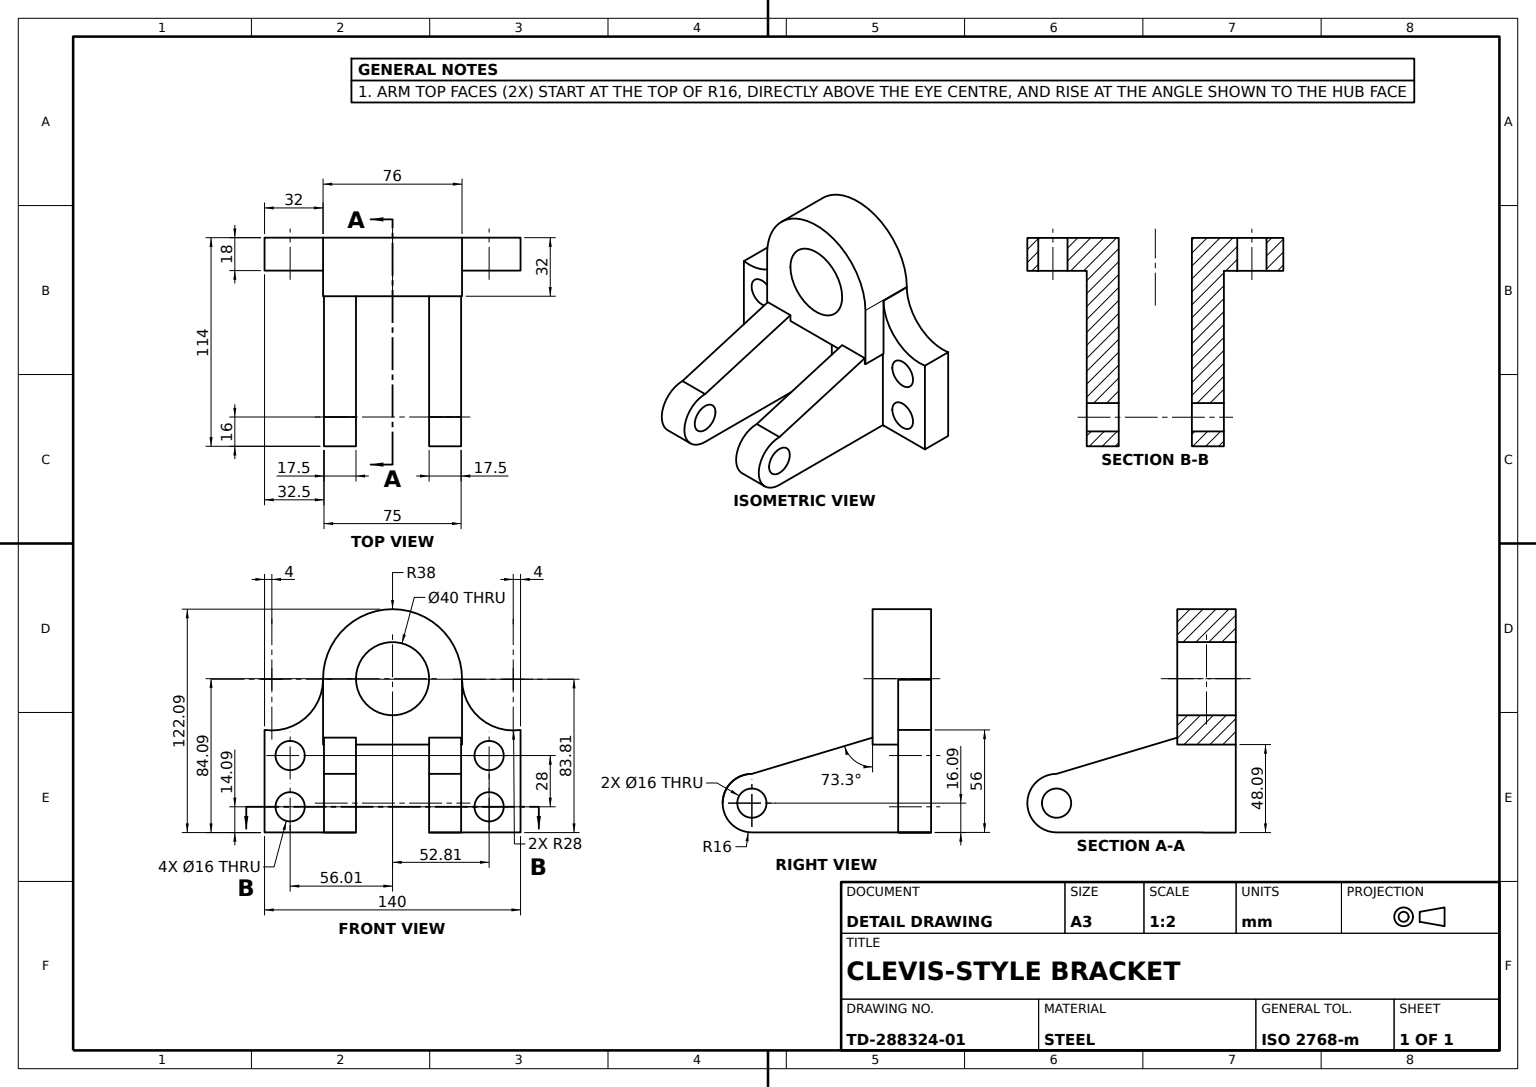
ISO-10303-21;
HEADER;
FILE_DESCRIPTION((''),'2;1');
FILE_NAME('','',(''),(''),'','','');
FILE_SCHEMA(('AUTOMOTIVE_DESIGN'));
ENDSEC;
DATA;
#1=APPLICATION_CONTEXT('');
#2=PRODUCT_CONTEXT('',#1,'mechanical');
#3=PRODUCT('','','',(#2));
#4=PRODUCT_DEFINITION_FORMATION('','',#3);
#5=PRODUCT_DEFINITION_CONTEXT('',#1,'design');
#6=PRODUCT_DEFINITION('','',#4,#5);
#7=PRODUCT_DEFINITION_SHAPE('','',#6);
#8=(LENGTH_UNIT()NAMED_UNIT(*)SI_UNIT(.MILLI.,.METRE.));
#9=(NAMED_UNIT(*)PLANE_ANGLE_UNIT()SI_UNIT($,.RADIAN.));
#10=(NAMED_UNIT(*)SI_UNIT($,.STERADIAN.)SOLID_ANGLE_UNIT());
#11=UNCERTAINTY_MEASURE_WITH_UNIT(LENGTH_MEASURE(1.E-05),#8,'distance_accuracy_value','');
#12=(GEOMETRIC_REPRESENTATION_CONTEXT(3)GLOBAL_UNCERTAINTY_ASSIGNED_CONTEXT((#11))GLOBAL_UNIT_ASSIGNED_CONTEXT((#8,#9,#10))REPRESENTATION_CONTEXT('',''));
#13=CARTESIAN_POINT('',(-48.006496,-34.,0.));
#14=VERTEX_POINT('',#13);
#15=CARTESIAN_POINT('',(-64.006496,-34.,0.));
#16=VERTEX_POINT('',#15);
#17=CARTESIAN_POINT('',(-56.006496,-34.,0.));
#18=DIRECTION('',(0.,0.,1.));
#19=DIRECTION('',(1.,0.,0.));
#20=AXIS2_PLACEMENT_3D('',#17,#18,#19);
#21=CIRCLE('',#20,8.);
#22=EDGE_CURVE('',#14,#16,#21,.T.);
#23=ORIENTED_EDGE('',*,*,#22,.F.);
#24=CARTESIAN_POINT('',(-48.006496,-34.,18.));
#25=VERTEX_POINT('',#24);
#26=VECTOR('',#18,1000.);
#27=LINE('',#13,#26);
#28=EDGE_CURVE('',#14,#25,#27,.T.);
#29=ORIENTED_EDGE('',*,*,#28,.T.);
#30=CARTESIAN_POINT('',(-64.006496,-34.,18.));
#31=VERTEX_POINT('',#30);
#32=CARTESIAN_POINT('',(-56.006496,-34.,18.));
#33=AXIS2_PLACEMENT_3D('',#32,#18,#19);
#34=CIRCLE('',#33,8.);
#35=EDGE_CURVE('',#25,#31,#34,.T.);
#36=ORIENTED_EDGE('',*,*,#35,.T.);
#37=LINE('',#15,#26);
#38=EDGE_CURVE('',#16,#31,#37,.T.);
#39=ORIENTED_EDGE('',*,*,#38,.F.);
#40=EDGE_LOOP('',(#23,#29,#36,#39));
#41=FACE_OUTER_BOUND('',#40,.T.);
#42=CYLINDRICAL_SURFACE('',#20,8.);
#43=ADVANCED_FACE('',(#41),#42,.F.);
#44=CARTESIAN_POINT('',(20.,-48.,98.));
#45=VERTEX_POINT('',#44);
#46=CARTESIAN_POINT('',(20.,-48.,18.));
#47=VERTEX_POINT('',#46);
#48=CARTESIAN_POINT('',(20.,-48.,114.));
#49=DIRECTION('',(0.,0.,-1.));
#50=VECTOR('',#49,1000.);
#51=LINE('',#48,#50);
#52=EDGE_CURVE('',#45,#47,#51,.T.);
#53=ORIENTED_EDGE('',*,*,#52,.T.);
#54=CARTESIAN_POINT('',(37.5,-48.,18.));
#55=VERTEX_POINT('',#54);
#56=DIRECTION('',(-1.,0.,0.));
#57=VECTOR('',#56,1000.);
#58=LINE('',#54,#57);
#59=EDGE_CURVE('',#55,#47,#58,.T.);
#60=ORIENTED_EDGE('',*,*,#59,.F.);
#61=CARTESIAN_POINT('',(37.5,-48.,98.));
#62=VERTEX_POINT('',#61);
#63=CARTESIAN_POINT('',(37.5,-48.,0.));
#64=LINE('',#63,#26);
#65=EDGE_CURVE('',#55,#62,#64,.T.);
#66=ORIENTED_EDGE('',*,*,#65,.T.);
#67=LINE('',#61,#57);
#68=EDGE_CURVE('',#62,#45,#67,.T.);
#69=ORIENTED_EDGE('',*,*,#68,.T.);
#70=EDGE_LOOP('',(#53,#60,#66,#69));
#71=FACE_OUTER_BOUND('',#70,.T.);
#72=DIRECTION('',(0.,-1.,0.));
#73=AXIS2_PLACEMENT_3D('',#63,#72,#49);
#74=PLANE('',#73);
#75=ADVANCED_FACE('',(#71),#74,.T.);
#76=CARTESIAN_POINT('',(-20.,-32.,90.));
#77=VERTEX_POINT('',#76);
#78=CARTESIAN_POINT('',(-20.,-32.,106.));
#79=VERTEX_POINT('',#78);
#80=CARTESIAN_POINT('',(-20.,-32.,98.));
#81=AXIS2_PLACEMENT_3D('',#80,#56,#72);
#82=CIRCLE('',#81,8.);
#83=EDGE_CURVE('',#77,#79,#82,.T.);
#84=ORIENTED_EDGE('',*,*,#83,.F.);
#85=CARTESIAN_POINT('',(-37.5,-32.,90.));
#86=VERTEX_POINT('',#85);
#87=CARTESIAN_POINT('',(70.,-32.,90.));
#88=LINE('',#87,#57);
#89=EDGE_CURVE('',#77,#86,#88,.T.);
#90=ORIENTED_EDGE('',*,*,#89,.T.);
#91=CARTESIAN_POINT('',(-37.5,-32.,106.));
#92=VERTEX_POINT('',#91);
#93=CARTESIAN_POINT('',(-37.5,-32.,98.));
#94=AXIS2_PLACEMENT_3D('',#93,#56,#18);
#95=CIRCLE('',#94,8.);
#96=EDGE_CURVE('',#86,#92,#95,.T.);
#97=ORIENTED_EDGE('',*,*,#96,.T.);
#98=CARTESIAN_POINT('',(70.,-32.,106.));
#99=LINE('',#98,#57);
#100=EDGE_CURVE('',#79,#92,#99,.T.);
#101=ORIENTED_EDGE('',*,*,#100,.F.);
#102=EDGE_LOOP('',(#84,#90,#97,#101));
#103=FACE_OUTER_BOUND('',#102,.T.);
#104=CARTESIAN_POINT('',(70.,-32.,98.));
#105=AXIS2_PLACEMENT_3D('',#104,#56,#18);
#106=CYLINDRICAL_SURFACE('',#105,8.);
#107=ADVANCED_FACE('',(#103),#106,.F.);
#108=CARTESIAN_POINT('',(37.5,-32.,90.));
#109=VERTEX_POINT('',#108);
#110=CARTESIAN_POINT('',(37.5,-32.,106.));
#111=VERTEX_POINT('',#110);
#112=CARTESIAN_POINT('',(37.5,-32.,98.));
#113=AXIS2_PLACEMENT_3D('',#112,#19,#49);
#114=CIRCLE('',#113,8.);
#115=EDGE_CURVE('',#109,#111,#114,.T.);
#116=ORIENTED_EDGE('',*,*,#115,.F.);
#117=EDGE_CURVE('',#111,#109,#114,.T.);
#118=ORIENTED_EDGE('',*,*,#117,.F.);
#119=EDGE_LOOP('',(#116,#118));
#120=FACE_BOUND('',#119,.T.);
#121=ORIENTED_EDGE('',*,*,#65,.F.);
#122=CARTESIAN_POINT('',(37.5,0.,18.));
#123=VERTEX_POINT('',#122);
#124=VECTOR('',#72,1000.);
#125=LINE('',#122,#124);
#126=EDGE_CURVE('',#123,#55,#125,.T.);
#127=ORIENTED_EDGE('',*,*,#126,.F.);
#128=CARTESIAN_POINT('',(37.5,0.,32.));
#129=VERTEX_POINT('',#128);
#130=LINE('',#128,#50);
#131=EDGE_CURVE('',#129,#123,#130,.T.);
#132=ORIENTED_EDGE('',*,*,#131,.F.);
#133=CARTESIAN_POINT('',(37.5,3.8,32.));
#134=VERTEX_POINT('',#133);
#135=CARTESIAN_POINT('',(37.5,36.,32.));
#136=DIRECTION('',(0.,1.,0.));
#137=VECTOR('',#136,1000.);
#138=LINE('',#135,#137);
#139=EDGE_CURVE('',#129,#134,#138,.T.);
#140=ORIENTED_EDGE('',*,*,#139,.T.);
#141=CARTESIAN_POINT('',(37.5,-16.,98.));
#142=VERTEX_POINT('',#141);
#143=CARTESIAN_POINT('',(37.5,12.293578,3.688073));
#144=DIRECTION('',(0.,0.287347886,-0.957826285));
#145=VECTOR('',#144,1000.);
#146=LINE('',#143,#145);
#147=EDGE_CURVE('',#142,#134,#146,.T.);
#148=ORIENTED_EDGE('',*,*,#147,.F.);
#149=CARTESIAN_POINT('',(37.5,-32.,114.));
#150=VERTEX_POINT('',#149);
#151=CIRCLE('',#113,16.);
#152=EDGE_CURVE('',#142,#150,#151,.T.);
#153=ORIENTED_EDGE('',*,*,#152,.T.);
#154=EDGE_CURVE('',#150,#62,#151,.T.);
#155=ORIENTED_EDGE('',*,*,#154,.T.);
#156=EDGE_LOOP('',(#121,#127,#132,#140,#148,#153,#155));
#157=FACE_OUTER_BOUND('',#156,.T.);
#158=CARTESIAN_POINT('',(37.5,0.,0.));
#159=AXIS2_PLACEMENT_3D('',#158,#19,#49);
#160=PLANE('',#159);
#161=ADVANCED_FACE('',(#120,#157),#160,.T.);
#162=CARTESIAN_POINT('',(-38.,-48.092936,18.));
#163=VERTEX_POINT('',#162);
#164=CARTESIAN_POINT('',(-38.,-48.092936,0.));
#165=VERTEX_POINT('',#164);
#166=LINE('',#162,#50);
#167=EDGE_CURVE('',#163,#165,#166,.T.);
#168=ORIENTED_EDGE('',*,*,#167,.F.);
#169=CARTESIAN_POINT('',(-38.,-48.,18.));
#170=VERTEX_POINT('',#169);
#171=CARTESIAN_POINT('',(-38.,0.,18.));
#172=LINE('',#171,#124);
#173=EDGE_CURVE('',#170,#163,#172,.T.);
#174=ORIENTED_EDGE('',*,*,#173,.F.);
#175=CARTESIAN_POINT('',(-38.,-48.,0.));
#176=VERTEX_POINT('',#175);
#177=LINE('',#169,#50);
#178=EDGE_CURVE('',#170,#176,#177,.T.);
#179=ORIENTED_EDGE('',*,*,#178,.T.);
#180=CARTESIAN_POINT('',(-38.,0.,0.));
#181=LINE('',#180,#124);
#182=EDGE_CURVE('',#176,#165,#181,.T.);
#183=ORIENTED_EDGE('',*,*,#182,.T.);
#184=EDGE_LOOP('',(#168,#174,#179,#183));
#185=FACE_OUTER_BOUND('',#184,.T.);
#186=AXIS2_PLACEMENT_3D('',#171,#19,#49);
#187=PLANE('',#186);
#188=ADVANCED_FACE('',(#185),#187,.F.);
#189=CARTESIAN_POINT('',(20.,-16.,98.));
#190=VERTEX_POINT('',#189);
#191=LINE('',#141,#57);
#192=EDGE_CURVE('',#142,#190,#191,.T.);
#193=ORIENTED_EDGE('',*,*,#192,.T.);
#194=CARTESIAN_POINT('',(20.,-32.,114.));
#195=VERTEX_POINT('',#194);
#196=CARTESIAN_POINT('',(20.,-32.,98.));
#197=AXIS2_PLACEMENT_3D('',#196,#19,#49);
#198=CIRCLE('',#197,16.);
#199=EDGE_CURVE('',#190,#195,#198,.T.);
#200=ORIENTED_EDGE('',*,*,#199,.T.);
#201=LINE('',#149,#57);
#202=EDGE_CURVE('',#150,#195,#201,.T.);
#203=ORIENTED_EDGE('',*,*,#202,.F.);
#204=ORIENTED_EDGE('',*,*,#152,.F.);
#205=EDGE_LOOP('',(#193,#200,#203,#204));
#206=FACE_OUTER_BOUND('',#205,.T.);
#207=AXIS2_PLACEMENT_3D('',#112,#56,#18);
#208=CYLINDRICAL_SURFACE('',#207,16.);
#209=ADVANCED_FACE('',(#206),#208,.T.);
#210=CARTESIAN_POINT('',(-20.,-48.,98.));
#211=VERTEX_POINT('',#210);
#212=CARTESIAN_POINT('',(-20.,-32.,114.));
#213=VERTEX_POINT('',#212);
#214=AXIS2_PLACEMENT_3D('',#80,#56,#18);
#215=CIRCLE('',#214,16.);
#216=EDGE_CURVE('',#211,#213,#215,.T.);
#217=ORIENTED_EDGE('',*,*,#216,.T.);
#218=CARTESIAN_POINT('',(-37.5,-32.,114.));
#219=VERTEX_POINT('',#218);
#220=EDGE_CURVE('',#213,#219,#201,.T.);
#221=ORIENTED_EDGE('',*,*,#220,.T.);
#222=CARTESIAN_POINT('',(-37.5,-48.,98.));
#223=VERTEX_POINT('',#222);
#224=AXIS2_PLACEMENT_3D('',#93,#19,#49);
#225=CIRCLE('',#224,16.);
#226=EDGE_CURVE('',#219,#223,#225,.T.);
#227=ORIENTED_EDGE('',*,*,#226,.T.);
#228=EDGE_CURVE('',#211,#223,#67,.T.);
#229=ORIENTED_EDGE('',*,*,#228,.F.);
#230=EDGE_LOOP('',(#217,#221,#227,#229));
#231=FACE_OUTER_BOUND('',#230,.T.);
#232=ADVANCED_FACE('',(#231),#208,.T.);
#233=CARTESIAN_POINT('',(70.,-48.,18.));
#234=VERTEX_POINT('',#233);
#235=CARTESIAN_POINT('',(70.,-48.,0.));
#236=VERTEX_POINT('',#235);
#237=LINE('',#233,#50);
#238=EDGE_CURVE('',#234,#236,#237,.T.);
#239=ORIENTED_EDGE('',*,*,#238,.F.);
#240=CARTESIAN_POINT('',(38.,-48.,18.));
#241=VERTEX_POINT('',#240);
#242=CARTESIAN_POINT('',(0.,-48.,18.));
#243=VECTOR('',#19,1000.);
#244=LINE('',#242,#243);
#245=EDGE_CURVE('',#241,#234,#244,.T.);
#246=ORIENTED_EDGE('',*,*,#245,.F.);
#247=CARTESIAN_POINT('',(38.,-48.,0.));
#248=VERTEX_POINT('',#247);
#249=LINE('',#240,#50);
#250=EDGE_CURVE('',#241,#248,#249,.T.);
#251=ORIENTED_EDGE('',*,*,#250,.T.);
#252=CARTESIAN_POINT('',(0.,-48.,0.));
#253=LINE('',#252,#243);
#254=EDGE_CURVE('',#248,#236,#253,.T.);
#255=ORIENTED_EDGE('',*,*,#254,.T.);
#256=EDGE_LOOP('',(#239,#246,#251,#255));
#257=FACE_OUTER_BOUND('',#256,.T.);
#258=AXIS2_PLACEMENT_3D('',#242,#136,#56);
#259=PLANE('',#258);
#260=ADVANCED_FACE('',(#257),#259,.F.);
#261=ORIENTED_EDGE('',*,*,#238,.T.);
#262=CARTESIAN_POINT('',(70.,8.,0.));
#263=VERTEX_POINT('',#262);
#264=CARTESIAN_POINT('',(70.,0.,0.));
#265=LINE('',#264,#137);
#266=EDGE_CURVE('',#236,#263,#265,.T.);
#267=ORIENTED_EDGE('',*,*,#266,.T.);
#268=CARTESIAN_POINT('',(70.,8.,18.));
#269=VERTEX_POINT('',#268);
#270=LINE('',#268,#50);
#271=EDGE_CURVE('',#269,#263,#270,.T.);
#272=ORIENTED_EDGE('',*,*,#271,.F.);
#273=CARTESIAN_POINT('',(70.,0.,18.));
#274=LINE('',#273,#137);
#275=EDGE_CURVE('',#234,#269,#274,.T.);
#276=ORIENTED_EDGE('',*,*,#275,.F.);
#277=EDGE_LOOP('',(#261,#267,#272,#276));
#278=FACE_OUTER_BOUND('',#277,.T.);
#279=AXIS2_PLACEMENT_3D('',#273,#56,#18);
#280=PLANE('',#279);
#281=ADVANCED_FACE('',(#278),#280,.F.);
#282=CARTESIAN_POINT('',(60.812643,-6.,18.));
#283=VERTEX_POINT('',#282);
#284=CARTESIAN_POINT('',(44.812643,-6.,18.));
#285=VERTEX_POINT('',#284);
#286=CARTESIAN_POINT('',(52.812643,-6.,18.));
#287=AXIS2_PLACEMENT_3D('',#286,#18,#19);
#288=CIRCLE('',#287,8.);
#289=EDGE_CURVE('',#283,#285,#288,.T.);
#290=ORIENTED_EDGE('',*,*,#289,.T.);
#291=CARTESIAN_POINT('',(44.812643,-6.,0.));
#292=VERTEX_POINT('',#291);
#293=LINE('',#291,#26);
#294=EDGE_CURVE('',#292,#285,#293,.T.);
#295=ORIENTED_EDGE('',*,*,#294,.F.);
#296=CARTESIAN_POINT('',(60.812643,-6.,0.));
#297=VERTEX_POINT('',#296);
#298=CARTESIAN_POINT('',(52.812643,-6.,0.));
#299=AXIS2_PLACEMENT_3D('',#298,#18,#19);
#300=CIRCLE('',#299,8.);
#301=EDGE_CURVE('',#297,#292,#300,.T.);
#302=ORIENTED_EDGE('',*,*,#301,.F.);
#303=LINE('',#296,#26);
#304=EDGE_CURVE('',#297,#283,#303,.T.);
#305=ORIENTED_EDGE('',*,*,#304,.T.);
#306=EDGE_LOOP('',(#290,#295,#302,#305));
#307=FACE_OUTER_BOUND('',#306,.T.);
#308=CYLINDRICAL_SURFACE('',#299,8.);
#309=ADVANCED_FACE('',(#307),#308,.F.);
#310=CARTESIAN_POINT('',(-37.5,-16.,98.));
#311=VERTEX_POINT('',#310);
#312=CARTESIAN_POINT('',(-37.5,3.8,32.));
#313=VERTEX_POINT('',#312);
#314=CARTESIAN_POINT('',(-37.5,12.293578,3.688073));
#315=LINE('',#314,#145);
#316=EDGE_CURVE('',#311,#313,#315,.T.);
#317=ORIENTED_EDGE('',*,*,#316,.F.);
#318=CARTESIAN_POINT('',(-20.,-16.,98.));
#319=VERTEX_POINT('',#318);
#320=EDGE_CURVE('',#319,#311,#191,.T.);
#321=ORIENTED_EDGE('',*,*,#320,.F.);
#322=CARTESIAN_POINT('',(-20.,3.8,32.));
#323=VERTEX_POINT('',#322);
#324=CARTESIAN_POINT('',(-20.,12.293578,3.688073));
#325=DIRECTION('',(0.,-0.287347886,0.957826285));
#326=VECTOR('',#325,1000.);
#327=LINE('',#324,#326);
#328=EDGE_CURVE('',#323,#319,#327,.T.);
#329=ORIENTED_EDGE('',*,*,#328,.F.);
#330=CARTESIAN_POINT('',(0.,3.8,32.));
#331=LINE('',#330,#57);
#332=EDGE_CURVE('',#323,#313,#331,.T.);
#333=ORIENTED_EDGE('',*,*,#332,.T.);
#334=EDGE_LOOP('',(#317,#321,#329,#333));
#335=FACE_OUTER_BOUND('',#334,.T.);
#336=DIRECTION('',(0.,0.957826285,0.287347886));
#337=AXIS2_PLACEMENT_3D('',#143,#336,#325);
#338=PLANE('',#337);
#339=ADVANCED_FACE('',(#335),#338,.T.);
#340=ORIENTED_EDGE('',*,*,#320,.T.);
#341=EDGE_CURVE('',#311,#219,#225,.T.);
#342=ORIENTED_EDGE('',*,*,#341,.T.);
#343=ORIENTED_EDGE('',*,*,#220,.F.);
#344=EDGE_CURVE('',#213,#319,#215,.T.);
#345=ORIENTED_EDGE('',*,*,#344,.T.);
#346=EDGE_LOOP('',(#340,#342,#343,#345));
#347=FACE_OUTER_BOUND('',#346,.T.);
#348=ADVANCED_FACE('',(#347),#208,.T.);
#349=CARTESIAN_POINT('',(38.,0.,32.));
#350=VERTEX_POINT('',#349);
#351=CARTESIAN_POINT('',(38.,0.,18.));
#352=VERTEX_POINT('',#351);
#353=LINE('',#349,#50);
#354=EDGE_CURVE('',#350,#352,#353,.T.);
#355=ORIENTED_EDGE('',*,*,#354,.T.);
#356=CARTESIAN_POINT('',(38.,35.4252,18.));
#357=VERTEX_POINT('',#356);
#358=LINE('',#351,#124);
#359=EDGE_CURVE('',#357,#352,#358,.T.);
#360=ORIENTED_EDGE('',*,*,#359,.F.);
#361=CARTESIAN_POINT('',(38.,35.4252,0.));
#362=VERTEX_POINT('',#361);
#363=LINE('',#356,#50);
#364=EDGE_CURVE('',#357,#362,#363,.T.);
#365=ORIENTED_EDGE('',*,*,#364,.T.);
#366=CARTESIAN_POINT('',(38.,36.,0.));
#367=VERTEX_POINT('',#366);
#368=CARTESIAN_POINT('',(38.,0.,0.));
#369=LINE('',#368,#137);
#370=EDGE_CURVE('',#362,#367,#369,.T.);
#371=ORIENTED_EDGE('',*,*,#370,.T.);
#372=CARTESIAN_POINT('',(38.,36.,32.));
#373=VERTEX_POINT('',#372);
#374=LINE('',#372,#50);
#375=EDGE_CURVE('',#373,#367,#374,.T.);
#376=ORIENTED_EDGE('',*,*,#375,.F.);
#377=LINE('',#349,#137);
#378=EDGE_CURVE('',#350,#373,#377,.T.);
#379=ORIENTED_EDGE('',*,*,#378,.F.);
#380=EDGE_LOOP('',(#355,#360,#365,#371,#376,#379));
#381=FACE_OUTER_BOUND('',#380,.T.);
#382=AXIS2_PLACEMENT_3D('',#349,#56,#72);
#383=PLANE('',#382);
#384=ADVANCED_FACE('',(#381),#383,.F.);
#385=LINE('',#351,#57);
#386=EDGE_CURVE('',#352,#123,#385,.T.);
#387=ORIENTED_EDGE('',*,*,#386,.T.);
#388=ORIENTED_EDGE('',*,*,#126,.T.);
#389=ORIENTED_EDGE('',*,*,#59,.T.);
#390=CARTESIAN_POINT('',(20.,-48.092936,18.));
#391=VERTEX_POINT('',#390);
#392=CARTESIAN_POINT('',(20.,0.,18.));
#393=LINE('',#392,#124);
#394=EDGE_CURVE('',#47,#391,#393,.T.);
#395=ORIENTED_EDGE('',*,*,#394,.T.);
#396=CARTESIAN_POINT('',(38.,-48.092936,18.));
#397=VERTEX_POINT('',#396);
#398=LINE('',#396,#243);
#399=EDGE_CURVE('',#391,#397,#398,.T.);
#400=ORIENTED_EDGE('',*,*,#399,.T.);
#401=LINE('',#351,#137);
#402=EDGE_CURVE('',#397,#241,#401,.T.);
#403=ORIENTED_EDGE('',*,*,#402,.T.);
#404=ORIENTED_EDGE('',*,*,#245,.T.);
#405=ORIENTED_EDGE('',*,*,#275,.T.);
#406=CARTESIAN_POINT('',(65.998525,35.7126,18.));
#407=AXIS2_PLACEMENT_3D('',#406,#49,#19);
#408=CIRCLE('',#407,28.);
#409=EDGE_CURVE('',#269,#357,#408,.T.);
#410=ORIENTED_EDGE('',*,*,#409,.T.);
#411=ORIENTED_EDGE('',*,*,#359,.T.);
#412=EDGE_LOOP('',(#387,#388,#389,#395,#400,#403,#404,#405,#410,#411));
#413=FACE_OUTER_BOUND('',#412,.T.);
#414=EDGE_CURVE('',#285,#283,#288,.T.);
#415=ORIENTED_EDGE('',*,*,#414,.F.);
#416=ORIENTED_EDGE('',*,*,#289,.F.);
#417=EDGE_LOOP('',(#415,#416));
#418=FACE_BOUND('',#417,.T.);
#419=CARTESIAN_POINT('',(60.812643,-34.,18.));
#420=VERTEX_POINT('',#419);
#421=CARTESIAN_POINT('',(44.812643,-34.,18.));
#422=VERTEX_POINT('',#421);
#423=CARTESIAN_POINT('',(52.812643,-34.,18.));
#424=AXIS2_PLACEMENT_3D('',#423,#18,#19);
#425=CIRCLE('',#424,8.);
#426=EDGE_CURVE('',#420,#422,#425,.T.);
#427=ORIENTED_EDGE('',*,*,#426,.F.);
#428=EDGE_CURVE('',#422,#420,#425,.T.);
#429=ORIENTED_EDGE('',*,*,#428,.F.);
#430=EDGE_LOOP('',(#427,#429));
#431=FACE_BOUND('',#430,.T.);
#432=CARTESIAN_POINT('',(0.,0.,18.));
#433=AXIS2_PLACEMENT_3D('',#432,#18,#19);
#434=PLANE('',#433);
#435=ADVANCED_FACE('',(#413,#418,#431),#434,.T.);
#436=CARTESIAN_POINT('',(65.998525,35.7126,0.));
#437=AXIS2_PLACEMENT_3D('',#436,#49,#19);
#438=CIRCLE('',#437,28.);
#439=EDGE_CURVE('',#263,#362,#438,.T.);
#440=ORIENTED_EDGE('',*,*,#439,.T.);
#441=ORIENTED_EDGE('',*,*,#364,.F.);
#442=ORIENTED_EDGE('',*,*,#409,.F.);
#443=ORIENTED_EDGE('',*,*,#271,.T.);
#444=EDGE_LOOP('',(#440,#441,#442,#443));
#445=FACE_OUTER_BOUND('',#444,.T.);
#446=AXIS2_PLACEMENT_3D('',#406,#49,#56);
#447=CYLINDRICAL_SURFACE('',#446,28.);
#448=ADVANCED_FACE('',(#445),#447,.F.);
#449=CARTESIAN_POINT('',(20.,3.8,32.));
#450=VERTEX_POINT('',#449);
#451=CARTESIAN_POINT('',(20.,12.293578,3.688073));
#452=LINE('',#451,#145);
#453=EDGE_CURVE('',#190,#450,#452,.T.);
#454=ORIENTED_EDGE('',*,*,#453,.F.);
#455=ORIENTED_EDGE('',*,*,#192,.F.);
#456=ORIENTED_EDGE('',*,*,#147,.T.);
#457=EDGE_CURVE('',#134,#450,#331,.T.);
#458=ORIENTED_EDGE('',*,*,#457,.T.);
#459=EDGE_LOOP('',(#454,#455,#456,#458));
#460=FACE_OUTER_BOUND('',#459,.T.);
#461=ADVANCED_FACE('',(#460),#338,.T.);
#462=CARTESIAN_POINT('',(20.,36.,32.));
#463=VERTEX_POINT('',#462);
#464=CARTESIAN_POINT('',(-20.,36.,32.));
#465=VERTEX_POINT('',#464);
#466=CARTESIAN_POINT('',(0.,36.,32.));
#467=AXIS2_PLACEMENT_3D('',#466,#18,#19);
#468=CIRCLE('',#467,20.);
#469=EDGE_CURVE('',#463,#465,#468,.T.);
#470=ORIENTED_EDGE('',*,*,#469,.T.);
#471=CARTESIAN_POINT('',(-20.,36.,0.));
#472=VERTEX_POINT('',#471);
#473=LINE('',#464,#50);
#474=EDGE_CURVE('',#465,#472,#473,.T.);
#475=ORIENTED_EDGE('',*,*,#474,.T.);
#476=CARTESIAN_POINT('',(20.,36.,0.));
#477=VERTEX_POINT('',#476);
#478=CARTESIAN_POINT('',(0.,36.,0.));
#479=AXIS2_PLACEMENT_3D('',#478,#18,#19);
#480=CIRCLE('',#479,20.);
#481=EDGE_CURVE('',#477,#472,#480,.T.);
#482=ORIENTED_EDGE('',*,*,#481,.F.);
#483=LINE('',#462,#50);
#484=EDGE_CURVE('',#463,#477,#483,.T.);
#485=ORIENTED_EDGE('',*,*,#484,.F.);
#486=EDGE_LOOP('',(#470,#475,#482,#485));
#487=FACE_OUTER_BOUND('',#486,.T.);
#488=AXIS2_PLACEMENT_3D('',#466,#49,#56);
#489=CYLINDRICAL_SURFACE('',#488,20.);
#490=ADVANCED_FACE('',(#487),#489,.F.);
#491=ORIENTED_EDGE('',*,*,#426,.T.);
#492=CARTESIAN_POINT('',(44.812643,-34.,0.));
#493=VERTEX_POINT('',#492);
#494=LINE('',#492,#26);
#495=EDGE_CURVE('',#493,#422,#494,.T.);
#496=ORIENTED_EDGE('',*,*,#495,.F.);
#497=CARTESIAN_POINT('',(60.812643,-34.,0.));
#498=VERTEX_POINT('',#497);
#499=CARTESIAN_POINT('',(52.812643,-34.,0.));
#500=AXIS2_PLACEMENT_3D('',#499,#18,#19);
#501=CIRCLE('',#500,8.);
#502=EDGE_CURVE('',#498,#493,#501,.T.);
#503=ORIENTED_EDGE('',*,*,#502,.F.);
#504=LINE('',#497,#26);
#505=EDGE_CURVE('',#498,#420,#504,.T.);
#506=ORIENTED_EDGE('',*,*,#505,.T.);
#507=EDGE_LOOP('',(#491,#496,#503,#506));
#508=FACE_OUTER_BOUND('',#507,.T.);
#509=CYLINDRICAL_SURFACE('',#500,8.);
#510=ADVANCED_FACE('',(#508),#509,.F.);
#511=EDGE_CURVE('',#195,#45,#198,.T.);
#512=ORIENTED_EDGE('',*,*,#511,.F.);
#513=ORIENTED_EDGE('',*,*,#199,.F.);
#514=ORIENTED_EDGE('',*,*,#453,.T.);
#515=CARTESIAN_POINT('',(20.,0.,32.));
#516=VERTEX_POINT('',#515);
#517=CARTESIAN_POINT('',(20.,74.,32.));
#518=LINE('',#517,#124);
#519=EDGE_CURVE('',#450,#516,#518,.T.);
#520=ORIENTED_EDGE('',*,*,#519,.T.);
#521=CARTESIAN_POINT('',(20.,0.,0.));
#522=VERTEX_POINT('',#521);
#523=LINE('',#392,#50);
#524=EDGE_CURVE('',#516,#522,#523,.T.);
#525=ORIENTED_EDGE('',*,*,#524,.T.);
#526=CARTESIAN_POINT('',(20.,-48.092936,0.));
#527=VERTEX_POINT('',#526);
#528=LINE('',#521,#124);
#529=EDGE_CURVE('',#522,#527,#528,.T.);
#530=ORIENTED_EDGE('',*,*,#529,.T.);
#531=LINE('',#390,#50);
#532=EDGE_CURVE('',#391,#527,#531,.T.);
#533=ORIENTED_EDGE('',*,*,#532,.F.);
#534=ORIENTED_EDGE('',*,*,#394,.F.);
#535=ORIENTED_EDGE('',*,*,#52,.F.);
#536=EDGE_LOOP('',(#512,#513,#514,#520,#525,#530,#533,#534,#535));
#537=FACE_OUTER_BOUND('',#536,.T.);
#538=CARTESIAN_POINT('',(20.,-32.,90.));
#539=VERTEX_POINT('',#538);
#540=CARTESIAN_POINT('',(20.,-32.,106.));
#541=VERTEX_POINT('',#540);
#542=AXIS2_PLACEMENT_3D('',#196,#19,#136);
#543=CIRCLE('',#542,8.);
#544=EDGE_CURVE('',#539,#541,#543,.T.);
#545=ORIENTED_EDGE('',*,*,#544,.T.);
#546=EDGE_CURVE('',#541,#539,#543,.T.);
#547=ORIENTED_EDGE('',*,*,#546,.T.);
#548=EDGE_LOOP('',(#545,#547));
#549=FACE_BOUND('',#548,.T.);
#550=AXIS2_PLACEMENT_3D('',#392,#19,#136);
#551=PLANE('',#550);
#552=ADVANCED_FACE('',(#537,#549),#551,.F.);
#553=CARTESIAN_POINT('',(-20.,-48.,18.));
#554=VERTEX_POINT('',#553);
#555=CARTESIAN_POINT('',(-37.5,-48.,18.));
#556=VERTEX_POINT('',#555);
#557=EDGE_CURVE('',#554,#556,#58,.T.);
#558=ORIENTED_EDGE('',*,*,#557,.F.);
#559=CARTESIAN_POINT('',(-20.,-48.,114.));
#560=LINE('',#559,#50);
#561=EDGE_CURVE('',#211,#554,#560,.T.);
#562=ORIENTED_EDGE('',*,*,#561,.F.);
#563=ORIENTED_EDGE('',*,*,#228,.T.);
#564=CARTESIAN_POINT('',(-37.5,-48.,0.));
#565=LINE('',#564,#26);
#566=EDGE_CURVE('',#556,#223,#565,.T.);
#567=ORIENTED_EDGE('',*,*,#566,.F.);
#568=EDGE_LOOP('',(#558,#562,#563,#567));
#569=FACE_OUTER_BOUND('',#568,.T.);
#570=ADVANCED_FACE('',(#569),#74,.T.);
#571=CARTESIAN_POINT('',(-70.,-48.,0.));
#572=VERTEX_POINT('',#571);
#573=LINE('',#252,#57);
#574=EDGE_CURVE('',#176,#572,#573,.T.);
#575=ORIENTED_EDGE('',*,*,#574,.F.);
#576=ORIENTED_EDGE('',*,*,#178,.F.);
#577=CARTESIAN_POINT('',(-70.,-48.,18.));
#578=VERTEX_POINT('',#577);
#579=LINE('',#242,#57);
#580=EDGE_CURVE('',#170,#578,#579,.T.);
#581=ORIENTED_EDGE('',*,*,#580,.T.);
#582=LINE('',#577,#50);
#583=EDGE_CURVE('',#578,#572,#582,.T.);
#584=ORIENTED_EDGE('',*,*,#583,.T.);
#585=EDGE_LOOP('',(#575,#576,#581,#584));
#586=FACE_OUTER_BOUND('',#585,.T.);
#587=AXIS2_PLACEMENT_3D('',#242,#72,#19);
#588=PLANE('',#587);
#589=ADVANCED_FACE('',(#586),#588,.T.);
#590=EDGE_CURVE('',#79,#77,#82,.T.);
#591=ORIENTED_EDGE('',*,*,#590,.F.);
#592=ORIENTED_EDGE('',*,*,#100,.T.);
#593=EDGE_CURVE('',#92,#86,#95,.T.);
#594=ORIENTED_EDGE('',*,*,#593,.T.);
#595=ORIENTED_EDGE('',*,*,#89,.F.);
#596=EDGE_LOOP('',(#591,#592,#594,#595));
#597=FACE_OUTER_BOUND('',#596,.T.);
#598=ADVANCED_FACE('',(#597),#106,.F.);
#599=ORIENTED_EDGE('',*,*,#583,.F.);
#600=CARTESIAN_POINT('',(-70.,8.,18.));
#601=VERTEX_POINT('',#600);
#602=CARTESIAN_POINT('',(-70.,0.,18.));
#603=LINE('',#602,#137);
#604=EDGE_CURVE('',#578,#601,#603,.T.);
#605=ORIENTED_EDGE('',*,*,#604,.T.);
#606=CARTESIAN_POINT('',(-70.,8.,0.));
#607=VERTEX_POINT('',#606);
#608=LINE('',#600,#50);
#609=EDGE_CURVE('',#601,#607,#608,.T.);
#610=ORIENTED_EDGE('',*,*,#609,.T.);
#611=CARTESIAN_POINT('',(-70.,0.,0.));
#612=LINE('',#611,#137);
#613=EDGE_CURVE('',#572,#607,#612,.T.);
#614=ORIENTED_EDGE('',*,*,#613,.F.);
#615=EDGE_LOOP('',(#599,#605,#610,#614));
#616=FACE_OUTER_BOUND('',#615,.T.);
#617=AXIS2_PLACEMENT_3D('',#602,#56,#18);
#618=PLANE('',#617);
#619=ADVANCED_FACE('',(#616),#618,.T.);
#620=ORIENTED_EDGE('',*,*,#505,.F.);
#621=EDGE_CURVE('',#493,#498,#501,.T.);
#622=ORIENTED_EDGE('',*,*,#621,.F.);
#623=ORIENTED_EDGE('',*,*,#495,.T.);
#624=ORIENTED_EDGE('',*,*,#428,.T.);
#625=EDGE_LOOP('',(#620,#622,#623,#624));
#626=FACE_OUTER_BOUND('',#625,.T.);
#627=ADVANCED_FACE('',(#626),#509,.F.);
#628=EDGE_CURVE('',#31,#25,#34,.T.);
#629=ORIENTED_EDGE('',*,*,#628,.T.);
#630=ORIENTED_EDGE('',*,*,#28,.F.);
#631=EDGE_CURVE('',#16,#14,#21,.T.);
#632=ORIENTED_EDGE('',*,*,#631,.F.);
#633=ORIENTED_EDGE('',*,*,#38,.T.);
#634=EDGE_LOOP('',(#629,#630,#632,#633));
#635=FACE_OUTER_BOUND('',#634,.T.);
#636=ADVANCED_FACE('',(#635),#42,.F.);
#637=CARTESIAN_POINT('',(-37.5,0.,32.));
#638=VERTEX_POINT('',#637);
#639=CARTESIAN_POINT('',(-37.5,0.,18.));
#640=VERTEX_POINT('',#639);
#641=LINE('',#637,#50);
#642=EDGE_CURVE('',#638,#640,#641,.T.);
#643=ORIENTED_EDGE('',*,*,#642,.F.);
#644=CARTESIAN_POINT('',(-38.,0.,32.));
#645=VERTEX_POINT('',#644);
#646=LINE('',#644,#243);
#647=EDGE_CURVE('',#645,#638,#646,.T.);
#648=ORIENTED_EDGE('',*,*,#647,.F.);
#649=VERTEX_POINT('',#171);
#650=LINE('',#644,#50);
#651=EDGE_CURVE('',#645,#649,#650,.T.);
#652=ORIENTED_EDGE('',*,*,#651,.T.);
#653=LINE('',#171,#57);
#654=EDGE_CURVE('',#640,#649,#653,.T.);
#655=ORIENTED_EDGE('',*,*,#654,.F.);
#656=EDGE_LOOP('',(#643,#648,#652,#655));
#657=FACE_OUTER_BOUND('',#656,.T.);
#658=AXIS2_PLACEMENT_3D('',#644,#136,#18);
#659=PLANE('',#658);
#660=ADVANCED_FACE('',(#657),#659,.F.);
#661=CARTESIAN_POINT('',(-38.,36.,0.));
#662=VERTEX_POINT('',#661);
#663=CIRCLE('',#479,38.);
#664=EDGE_CURVE('',#367,#662,#663,.T.);
#665=ORIENTED_EDGE('',*,*,#664,.T.);
#666=CARTESIAN_POINT('',(-38.,36.,32.));
#667=VERTEX_POINT('',#666);
#668=LINE('',#666,#50);
#669=EDGE_CURVE('',#667,#662,#668,.T.);
#670=ORIENTED_EDGE('',*,*,#669,.F.);
#671=CIRCLE('',#467,38.);
#672=EDGE_CURVE('',#373,#667,#671,.T.);
#673=ORIENTED_EDGE('',*,*,#672,.F.);
#674=ORIENTED_EDGE('',*,*,#375,.T.);
#675=EDGE_LOOP('',(#665,#670,#673,#674));
#676=FACE_OUTER_BOUND('',#675,.T.);
#677=CYLINDRICAL_SURFACE('',#488,38.);
#678=ADVANCED_FACE('',(#676),#677,.T.);
#679=ORIENTED_EDGE('',*,*,#593,.F.);
#680=ORIENTED_EDGE('',*,*,#96,.F.);
#681=EDGE_LOOP('',(#679,#680));
#682=FACE_BOUND('',#681,.T.);
#683=ORIENTED_EDGE('',*,*,#226,.F.);
#684=ORIENTED_EDGE('',*,*,#341,.F.);
#685=ORIENTED_EDGE('',*,*,#316,.T.);
#686=CARTESIAN_POINT('',(-37.5,36.,32.));
#687=LINE('',#686,#137);
#688=EDGE_CURVE('',#638,#313,#687,.T.);
#689=ORIENTED_EDGE('',*,*,#688,.F.);
#690=ORIENTED_EDGE('',*,*,#642,.T.);
#691=LINE('',#639,#124);
#692=EDGE_CURVE('',#640,#556,#691,.T.);
#693=ORIENTED_EDGE('',*,*,#692,.T.);
#694=ORIENTED_EDGE('',*,*,#566,.T.);
#695=EDGE_LOOP('',(#683,#684,#685,#689,#690,#693,#694));
#696=FACE_OUTER_BOUND('',#695,.T.);
#697=CARTESIAN_POINT('',(-37.5,0.,0.));
#698=AXIS2_PLACEMENT_3D('',#697,#19,#49);
#699=PLANE('',#698);
#700=ADVANCED_FACE('',(#682,#696),#699,.F.);
#701=ORIENTED_EDGE('',*,*,#621,.T.);
#702=ORIENTED_EDGE('',*,*,#502,.T.);
#703=EDGE_LOOP('',(#701,#702));
#704=FACE_BOUND('',#703,.T.);
#705=ORIENTED_EDGE('',*,*,#481,.T.);
#706=EDGE_CURVE('',#472,#477,#480,.T.);
#707=ORIENTED_EDGE('',*,*,#706,.T.);
#708=EDGE_LOOP('',(#705,#707));
#709=FACE_BOUND('',#708,.T.);
#710=ORIENTED_EDGE('',*,*,#22,.T.);
#711=ORIENTED_EDGE('',*,*,#631,.T.);
#712=EDGE_LOOP('',(#710,#711));
#713=FACE_BOUND('',#712,.T.);
#714=CARTESIAN_POINT('',(-64.006496,-6.,0.));
#715=VERTEX_POINT('',#714);
#716=CARTESIAN_POINT('',(-48.006496,-6.,0.));
#717=VERTEX_POINT('',#716);
#718=CARTESIAN_POINT('',(-56.006496,-6.,0.));
#719=AXIS2_PLACEMENT_3D('',#718,#18,#19);
#720=CIRCLE('',#719,8.);
#721=EDGE_CURVE('',#715,#717,#720,.T.);
#722=ORIENTED_EDGE('',*,*,#721,.T.);
#723=EDGE_CURVE('',#717,#715,#720,.T.);
#724=ORIENTED_EDGE('',*,*,#723,.T.);
#725=EDGE_LOOP('',(#722,#724));
#726=FACE_BOUND('',#725,.T.);
#727=EDGE_CURVE('',#292,#297,#300,.T.);
#728=ORIENTED_EDGE('',*,*,#727,.T.);
#729=ORIENTED_EDGE('',*,*,#301,.T.);
#730=EDGE_LOOP('',(#728,#729));
#731=FACE_BOUND('',#730,.T.);
#732=CARTESIAN_POINT('',(38.,-48.092936,0.));
#733=VERTEX_POINT('',#732);
#734=EDGE_CURVE('',#733,#248,#369,.T.);
#735=ORIENTED_EDGE('',*,*,#734,.F.);
#736=LINE('',#732,#243);
#737=EDGE_CURVE('',#527,#733,#736,.T.);
#738=ORIENTED_EDGE('',*,*,#737,.F.);
#739=ORIENTED_EDGE('',*,*,#529,.F.);
#740=CARTESIAN_POINT('',(-20.,0.,0.));
#741=VERTEX_POINT('',#740);
#742=LINE('',#180,#243);
#743=EDGE_CURVE('',#741,#522,#742,.T.);
#744=ORIENTED_EDGE('',*,*,#743,.F.);
#745=CARTESIAN_POINT('',(-20.,-48.092936,0.));
#746=VERTEX_POINT('',#745);
#747=LINE('',#740,#137);
#748=EDGE_CURVE('',#746,#741,#747,.T.);
#749=ORIENTED_EDGE('',*,*,#748,.F.);
#750=LINE('',#164,#243);
#751=EDGE_CURVE('',#165,#746,#750,.T.);
#752=ORIENTED_EDGE('',*,*,#751,.F.);
#753=ORIENTED_EDGE('',*,*,#182,.F.);
#754=ORIENTED_EDGE('',*,*,#574,.T.);
#755=ORIENTED_EDGE('',*,*,#613,.T.);
#756=CARTESIAN_POINT('',(-38.,35.4252,0.));
#757=VERTEX_POINT('',#756);
#758=CARTESIAN_POINT('',(-65.998525,35.7126,0.));
#759=AXIS2_PLACEMENT_3D('',#758,#18,#19);
#760=CIRCLE('',#759,28.);
#761=EDGE_CURVE('',#607,#757,#760,.T.);
#762=ORIENTED_EDGE('',*,*,#761,.T.);
#763=LINE('',#661,#124);
#764=EDGE_CURVE('',#662,#757,#763,.T.);
#765=ORIENTED_EDGE('',*,*,#764,.F.);
#766=ORIENTED_EDGE('',*,*,#664,.F.);
#767=ORIENTED_EDGE('',*,*,#370,.F.);
#768=ORIENTED_EDGE('',*,*,#439,.F.);
#769=ORIENTED_EDGE('',*,*,#266,.F.);
#770=ORIENTED_EDGE('',*,*,#254,.F.);
#771=EDGE_LOOP('',(#735,#738,#739,#744,#749,#752,#753,#754,#755,#762,#765,#766,#767,#768,#769,#770));
#772=FACE_OUTER_BOUND('',#771,.T.);
#773=PLANE('',#479);
#774=ADVANCED_FACE('',(#704,#709,#713,#726,#731,#772),#773,.F.);
#775=CARTESIAN_POINT('',(-64.006496,-6.,18.));
#776=VERTEX_POINT('',#775);
#777=CARTESIAN_POINT('',(-48.006496,-6.,18.));
#778=VERTEX_POINT('',#777);
#779=CARTESIAN_POINT('',(-56.006496,-6.,18.));
#780=AXIS2_PLACEMENT_3D('',#779,#18,#19);
#781=CIRCLE('',#780,8.);
#782=EDGE_CURVE('',#776,#778,#781,.T.);
#783=ORIENTED_EDGE('',*,*,#782,.T.);
#784=LINE('',#716,#26);
#785=EDGE_CURVE('',#717,#778,#784,.T.);
#786=ORIENTED_EDGE('',*,*,#785,.F.);
#787=ORIENTED_EDGE('',*,*,#721,.F.);
#788=LINE('',#714,#26);
#789=EDGE_CURVE('',#715,#776,#788,.T.);
#790=ORIENTED_EDGE('',*,*,#789,.T.);
#791=EDGE_LOOP('',(#783,#786,#787,#790));
#792=FACE_OUTER_BOUND('',#791,.T.);
#793=CYLINDRICAL_SURFACE('',#719,8.);
#794=ADVANCED_FACE('',(#792),#793,.F.);
#795=ORIENTED_EDGE('',*,*,#532,.T.);
#796=ORIENTED_EDGE('',*,*,#737,.T.);
#797=LINE('',#396,#50);
#798=EDGE_CURVE('',#397,#733,#797,.T.);
#799=ORIENTED_EDGE('',*,*,#798,.F.);
#800=ORIENTED_EDGE('',*,*,#399,.F.);
#801=EDGE_LOOP('',(#795,#796,#799,#800));
#802=FACE_OUTER_BOUND('',#801,.T.);
#803=AXIS2_PLACEMENT_3D('',#396,#136,#18);
#804=PLANE('',#803);
#805=ADVANCED_FACE('',(#802),#804,.F.);
#806=CARTESIAN_POINT('',(-20.,-48.092936,18.));
#807=VERTEX_POINT('',#806);
#808=LINE('',#806,#50);
#809=EDGE_CURVE('',#807,#746,#808,.T.);
#810=ORIENTED_EDGE('',*,*,#809,.T.);
#811=ORIENTED_EDGE('',*,*,#748,.T.);
#812=CARTESIAN_POINT('',(-20.,0.,32.));
#813=VERTEX_POINT('',#812);
#814=CARTESIAN_POINT('',(-20.,0.,18.));
#815=LINE('',#814,#50);
#816=EDGE_CURVE('',#813,#741,#815,.T.);
#817=ORIENTED_EDGE('',*,*,#816,.F.);
#818=CARTESIAN_POINT('',(-20.,74.,32.));
#819=LINE('',#818,#124);
#820=EDGE_CURVE('',#323,#813,#819,.T.);
#821=ORIENTED_EDGE('',*,*,#820,.F.);
#822=ORIENTED_EDGE('',*,*,#328,.T.);
#823=ORIENTED_EDGE('',*,*,#344,.F.);
#824=ORIENTED_EDGE('',*,*,#216,.F.);
#825=ORIENTED_EDGE('',*,*,#561,.T.);
#826=LINE('',#814,#137);
#827=EDGE_CURVE('',#807,#554,#826,.T.);
#828=ORIENTED_EDGE('',*,*,#827,.F.);
#829=EDGE_LOOP('',(#810,#811,#817,#821,#822,#823,#824,#825,#828));
#830=FACE_OUTER_BOUND('',#829,.T.);
#831=ORIENTED_EDGE('',*,*,#83,.T.);
#832=ORIENTED_EDGE('',*,*,#590,.T.);
#833=EDGE_LOOP('',(#831,#832));
#834=FACE_BOUND('',#833,.T.);
#835=AXIS2_PLACEMENT_3D('',#814,#56,#72);
#836=PLANE('',#835);
#837=ADVANCED_FACE('',(#830,#834),#836,.F.);
#838=ORIENTED_EDGE('',*,*,#706,.F.);
#839=ORIENTED_EDGE('',*,*,#474,.F.);
#840=EDGE_CURVE('',#465,#463,#468,.T.);
#841=ORIENTED_EDGE('',*,*,#840,.T.);
#842=ORIENTED_EDGE('',*,*,#484,.T.);
#843=EDGE_LOOP('',(#838,#839,#841,#842));
#844=FACE_OUTER_BOUND('',#843,.T.);
#845=ADVANCED_FACE('',(#844),#489,.F.);
#846=ORIENTED_EDGE('',*,*,#609,.F.);
#847=CARTESIAN_POINT('',(-38.,35.4252,18.));
#848=VERTEX_POINT('',#847);
#849=CARTESIAN_POINT('',(-65.998525,35.7126,18.));
#850=AXIS2_PLACEMENT_3D('',#849,#18,#19);
#851=CIRCLE('',#850,28.);
#852=EDGE_CURVE('',#601,#848,#851,.T.);
#853=ORIENTED_EDGE('',*,*,#852,.T.);
#854=LINE('',#847,#50);
#855=EDGE_CURVE('',#848,#757,#854,.T.);
#856=ORIENTED_EDGE('',*,*,#855,.T.);
#857=ORIENTED_EDGE('',*,*,#761,.F.);
#858=EDGE_LOOP('',(#846,#853,#856,#857));
#859=FACE_OUTER_BOUND('',#858,.T.);
#860=AXIS2_PLACEMENT_3D('',#849,#49,#56);
#861=CYLINDRICAL_SURFACE('',#860,28.);
#862=ADVANCED_FACE('',(#859),#861,.F.);
#863=EDGE_CURVE('',#778,#776,#781,.T.);
#864=ORIENTED_EDGE('',*,*,#863,.T.);
#865=ORIENTED_EDGE('',*,*,#789,.F.);
#866=ORIENTED_EDGE('',*,*,#723,.F.);
#867=ORIENTED_EDGE('',*,*,#785,.T.);
#868=EDGE_LOOP('',(#864,#865,#866,#867));
#869=FACE_OUTER_BOUND('',#868,.T.);
#870=ADVANCED_FACE('',(#869),#793,.F.);
#871=ORIENTED_EDGE('',*,*,#692,.F.);
#872=ORIENTED_EDGE('',*,*,#654,.T.);
#873=EDGE_CURVE('',#848,#649,#172,.T.);
#874=ORIENTED_EDGE('',*,*,#873,.F.);
#875=ORIENTED_EDGE('',*,*,#852,.F.);
#876=ORIENTED_EDGE('',*,*,#604,.F.);
#877=ORIENTED_EDGE('',*,*,#580,.F.);
#878=ORIENTED_EDGE('',*,*,#173,.T.);
#879=LINE('',#162,#243);
#880=EDGE_CURVE('',#163,#807,#879,.T.);
#881=ORIENTED_EDGE('',*,*,#880,.T.);
#882=ORIENTED_EDGE('',*,*,#827,.T.);
#883=ORIENTED_EDGE('',*,*,#557,.T.);
#884=EDGE_LOOP('',(#871,#872,#874,#875,#876,#877,#878,#881,#882,#883));
#885=FACE_OUTER_BOUND('',#884,.T.);
#886=ORIENTED_EDGE('',*,*,#35,.F.);
#887=ORIENTED_EDGE('',*,*,#628,.F.);
#888=EDGE_LOOP('',(#886,#887));
#889=FACE_BOUND('',#888,.T.);
#890=ORIENTED_EDGE('',*,*,#782,.F.);
#891=ORIENTED_EDGE('',*,*,#863,.F.);
#892=EDGE_LOOP('',(#890,#891));
#893=FACE_BOUND('',#892,.T.);
#894=ADVANCED_FACE('',(#885,#889,#893),#434,.T.);
#895=ORIENTED_EDGE('',*,*,#743,.T.);
#896=ORIENTED_EDGE('',*,*,#524,.F.);
#897=CARTESIAN_POINT('',(0.,0.,32.));
#898=LINE('',#897,#57);
#899=EDGE_CURVE('',#516,#813,#898,.T.);
#900=ORIENTED_EDGE('',*,*,#899,.T.);
#901=ORIENTED_EDGE('',*,*,#816,.T.);
#902=EDGE_LOOP('',(#895,#896,#900,#901));
#903=FACE_OUTER_BOUND('',#902,.T.);
#904=ADVANCED_FACE('',(#903),#659,.F.);
#905=ORIENTED_EDGE('',*,*,#672,.T.);
#906=LINE('',#666,#124);
#907=EDGE_CURVE('',#667,#645,#906,.T.);
#908=ORIENTED_EDGE('',*,*,#907,.T.);
#909=ORIENTED_EDGE('',*,*,#647,.T.);
#910=ORIENTED_EDGE('',*,*,#688,.T.);
#911=ORIENTED_EDGE('',*,*,#332,.F.);
#912=ORIENTED_EDGE('',*,*,#820,.T.);
#913=ORIENTED_EDGE('',*,*,#899,.F.);
#914=ORIENTED_EDGE('',*,*,#519,.F.);
#915=ORIENTED_EDGE('',*,*,#457,.F.);
#916=ORIENTED_EDGE('',*,*,#139,.F.);
#917=EDGE_CURVE('',#129,#350,#646,.T.);
#918=ORIENTED_EDGE('',*,*,#917,.T.);
#919=ORIENTED_EDGE('',*,*,#378,.T.);
#920=EDGE_LOOP('',(#905,#908,#909,#910,#911,#912,#913,#914,#915,#916,#918,#919));
#921=FACE_OUTER_BOUND('',#920,.T.);
#922=ORIENTED_EDGE('',*,*,#469,.F.);
#923=ORIENTED_EDGE('',*,*,#840,.F.);
#924=EDGE_LOOP('',(#922,#923));
#925=FACE_BOUND('',#924,.T.);
#926=PLANE('',#467);
#927=ADVANCED_FACE('',(#921,#925),#926,.T.);
#928=ORIENTED_EDGE('',*,*,#167,.T.);
#929=ORIENTED_EDGE('',*,*,#751,.T.);
#930=ORIENTED_EDGE('',*,*,#809,.F.);
#931=ORIENTED_EDGE('',*,*,#880,.F.);
#932=EDGE_LOOP('',(#928,#929,#930,#931));
#933=FACE_OUTER_BOUND('',#932,.T.);
#934=AXIS2_PLACEMENT_3D('',#162,#136,#18);
#935=PLANE('',#934);
#936=ADVANCED_FACE('',(#933),#935,.F.);
#937=ORIENTED_EDGE('',*,*,#154,.F.);
#938=ORIENTED_EDGE('',*,*,#202,.T.);
#939=ORIENTED_EDGE('',*,*,#511,.T.);
#940=ORIENTED_EDGE('',*,*,#68,.F.);
#941=EDGE_LOOP('',(#937,#938,#939,#940));
#942=FACE_OUTER_BOUND('',#941,.T.);
#943=ADVANCED_FACE('',(#942),#208,.T.);
#944=ORIENTED_EDGE('',*,*,#727,.F.);
#945=ORIENTED_EDGE('',*,*,#294,.T.);
#946=ORIENTED_EDGE('',*,*,#414,.T.);
#947=ORIENTED_EDGE('',*,*,#304,.F.);
#948=EDGE_LOOP('',(#944,#945,#946,#947));
#949=FACE_OUTER_BOUND('',#948,.T.);
#950=ADVANCED_FACE('',(#949),#308,.F.);
#951=ORIENTED_EDGE('',*,*,#117,.T.);
#952=EDGE_CURVE('',#109,#539,#88,.T.);
#953=ORIENTED_EDGE('',*,*,#952,.T.);
#954=ORIENTED_EDGE('',*,*,#546,.F.);
#955=EDGE_CURVE('',#111,#541,#99,.T.);
#956=ORIENTED_EDGE('',*,*,#955,.F.);
#957=EDGE_LOOP('',(#951,#953,#954,#956));
#958=FACE_OUTER_BOUND('',#957,.T.);
#959=ADVANCED_FACE('',(#958),#106,.F.);
#960=ORIENTED_EDGE('',*,*,#354,.F.);
#961=ORIENTED_EDGE('',*,*,#917,.F.);
#962=ORIENTED_EDGE('',*,*,#131,.T.);
#963=ORIENTED_EDGE('',*,*,#386,.F.);
#964=EDGE_LOOP('',(#960,#961,#962,#963));
#965=FACE_OUTER_BOUND('',#964,.T.);
#966=ADVANCED_FACE('',(#965),#659,.F.);
#967=ORIENTED_EDGE('',*,*,#669,.T.);
#968=ORIENTED_EDGE('',*,*,#764,.T.);
#969=ORIENTED_EDGE('',*,*,#855,.F.);
#970=ORIENTED_EDGE('',*,*,#873,.T.);
#971=ORIENTED_EDGE('',*,*,#651,.F.);
#972=ORIENTED_EDGE('',*,*,#907,.F.);
#973=EDGE_LOOP('',(#967,#968,#969,#970,#971,#972));
#974=FACE_OUTER_BOUND('',#973,.T.);
#975=AXIS2_PLACEMENT_3D('',#666,#19,#49);
#976=PLANE('',#975);
#977=ADVANCED_FACE('',(#974),#976,.F.);
#978=ORIENTED_EDGE('',*,*,#250,.F.);
#979=ORIENTED_EDGE('',*,*,#402,.F.);
#980=ORIENTED_EDGE('',*,*,#798,.T.);
#981=ORIENTED_EDGE('',*,*,#734,.T.);
#982=EDGE_LOOP('',(#978,#979,#980,#981));
#983=FACE_OUTER_BOUND('',#982,.T.);
#984=AXIS2_PLACEMENT_3D('',#351,#56,#18);
#985=PLANE('',#984);
#986=ADVANCED_FACE('',(#983),#985,.F.);
#987=ORIENTED_EDGE('',*,*,#955,.T.);
#988=ORIENTED_EDGE('',*,*,#544,.F.);
#989=ORIENTED_EDGE('',*,*,#952,.F.);
#990=ORIENTED_EDGE('',*,*,#115,.T.);
#991=EDGE_LOOP('',(#987,#988,#989,#990));
#992=FACE_OUTER_BOUND('',#991,.T.);
#993=ADVANCED_FACE('',(#992),#106,.F.);
#994=CLOSED_SHELL('',(#43,#75,#107,#161,#188,#209,#232,#260,#281,#309,#339,#348,#384,#435,#448,#461,#490,#510,#552,#570,#589,#598,#619,#627,#636,#660,#678,#700,#774,#794,#805,#837,#845,#862,#870,#894,#904,#927,#936,#943,#950,#959,#966,#977,#986,#993));
#995=MANIFOLD_SOLID_BREP('',#994);
#996=ADVANCED_BREP_SHAPE_REPRESENTATION('',(#995),#12);
#997=SHAPE_DEFINITION_REPRESENTATION(#7,#996);
ENDSEC;
END-ISO-10303-21;
